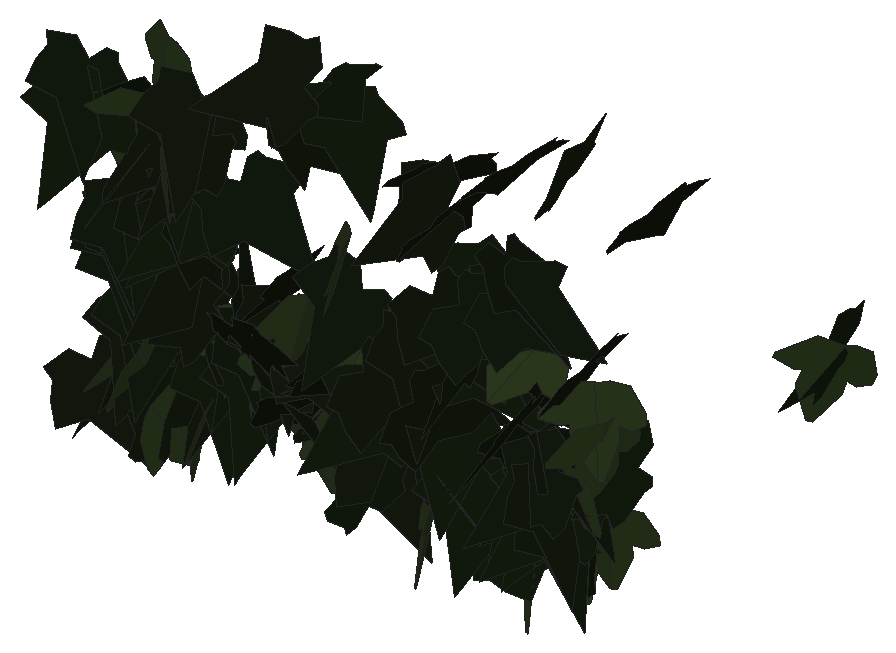
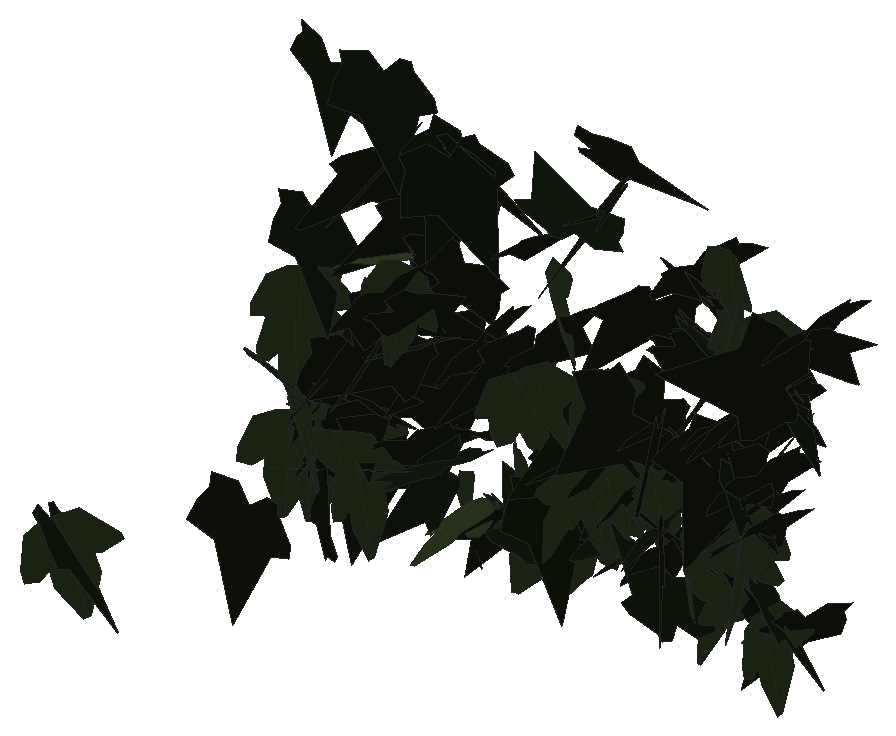
# SketchUp Ruby script. Lengths in inches.
U = 1.inch
M = Sketchup.active_model
def pt(a) = Geom::Point3d.new(a.map { |v| v * U })
def face(e, loops, mat)
  f = e.add_face(loops[0].map { |a| pt(a) })
  loops[1..].each { |l| e.add_face(l.map { |a| pt(a) }).erase! }
  f.material = f.back_material = mat if mat
  f
end
# faces: each face lists its corners as indices into pts; further lists are holes
def faces(e, pts, list, mat = nil) = list.each { |f| face(e, (f[0].is_a?(Array) ? f : [f]).map { |l| l.map { |i| pts[i] } }, mat) }
# xy, xz, yz: faces in a plane at the given z, y or x. An outline is a flat list of corners, or four numbers for a rectangle; further outlines are holes
def ring(l) = l.size == 4 ? [[l[0], l[1]], [l[2], l[1]], [l[2], l[3]], [l[0], l[3]]] : l.each_slice(2).to_a
def flat(e, list, mat, &to3) = list.each { |f| face(e, (f[0].is_a?(Array) ? f : [f]).map { |l| ring(l).map { |u, v| to3.(u, v) } }, mat) }
def xy(e, z, list, mat = nil) = flat(e, list, mat) { |x, y| [x, y, z] }
def xz(e, y, list, mat = nil) = flat(e, list, mat) { |x, z| [x, y, z] }
def yz(e, x, list, mat = nil) = flat(e, list, mat) { |y, z| [x, y, z] }
def lines(e, pts, list) = list.each { |a, b| e.add_line(pt(pts[a]), pt(pts[b])) }
# prism: a flat outline (further loops are holes) pulled along v
def prism(e, loops, v, mat = nil)
  f = face(e, loops, mat); d = Geom::Vector3d.new(v.map { |x| x * U })
  f.pushpull(f.normal.samedirection?(d) ? d.length : -d.length)
end
def box(e, o, s, mat = nil) = prism(e, [[o, [o[0] + s[0], o[1], o[2]], [o[0] + s[0], o[1] + s[1], o[2]], [o[0], o[1] + s[1], o[2]]]], [0, 0, s[2]], mat)
def at(x, y, z, deg = 0) = Geom::Transformation.translation(pt([x, y, z])) * Geom::Transformation.rotation(ORIGIN, Z_AXIS, deg.degrees)
def axes(o, x, y, z) = Geom::Transformation.new([*x, 0, *y, 0, *z, 0, *pt(o).to_a, 1])
def part(name) = M.definitions.add(name)
# library, detail: a bought-in or finely detailed component or shape, given as its bounding box
def library(name, o, s) = part(name).tap { |d| box(d.entities, o, s) }
def detail(e, o, s) = box(e.add_group.entities, o, s)
def put(e, d, t, mat = nil) = e.add_instance(d, t).tap { |i| i.material = mat if mat }
def group(e, t, mat = nil) = e.add_group.tap { |g| g.transformation = t; g.material = mat if mat }.entities
root = M.entities
M.materials.add("efeu1").color = [18, 25, 13]
M.materials.add("efeu2").color = [43, 57, 29]
c1 = part("ivyleaf_9")
p = [[1.54,2.16,1.25],[1.36,2.04,1.19],[-0.21,0.99,0.68],[-0.71,1.11,0.82],[-0.85,0.86,0.67],[-0.8,0.17,0.21],
  [-0.9,-0.01,0.1],[-0.67,-0.16,-0.02],[-0.08,-0.08,-0.05],[-0.03,-0.6,-0.4],[0.65,-0.88,-0.66],[0.83,-0.6,-0.49],
  [1.29,-0.42,-0.43],[1.8125,-0.07,-0.26],[1.21,0.44,0.15]]
faces(c1.entities,p,[[0,1,2,3,4,5,6,7,8,9,10,11,12,13,14]],"efeu1")
c2 = part("ivyleaf_10")
p = [[0,0.5,-0.03],[-0.0625,2.02,-0.43],[-0.19,2.01,-0.46],[-0.54,1.05,-0.29],[-0.52,0.625,-0.18],[-0.83,0.76,-0.28],
  [-1.16,0.64,-0.33],[-1.15,0.33,-0.24],[-0.77,-0.39,0.02],[-0.3,-0.51,0.16],[0.04,-0.48,0.23],[-0.02,2.01,-0.4375],
  [-0.06,2.01,-0.43],[0.04,-0.49,0.23],[0.67,-0.49,0.14],[1.38,0.36,-0.2],[1.375,0.51,-0.24],[0.81,0.65,-0.19],
  [0.62,0.59,-0.15],[0.6,1.09,-0.28],[0.5,1.23,-0.31]]
faces(c2.entities,p,[[0,1,2,3,4,5,6,7,8,9,10],[11,12,0,13,14,15,16,17,18,19,20]],"efeu2")
put(root,c1,axes([47.72,220.88,250.6],[0.48269,0.07432,-0.10717],[-0.10687,-0.01009,-0.48834],[-0.07475,0.49434,0.00615]))
put(root,c1,axes([45.87,221.22,251.43],[-0.28658,-0.25776,-0.31848],[0.28688,0.15125,-0.38056],[0.29252,-0.40085,0.0612]))
put(root,c1,axes([45.86,221,251.9],[-0.24087,0.43778,-0.01816],[0.00545,-0.01773,-0.49966],[-0.43813,-0.2409,0.00377]))
put(root,c1,axes([50.55,221.21,253.1],[-0.485,0.08676,0.08514],[-0.08165,0.02691,-0.49255],[-0.09005,-0.49168,-0.01194]))
put(root,c1,axes([46.95,221.31,252.72],[-0.48269,-0.01355,-0.12972],[0.13042,-0.04902,-0.4802],[0.0003,-0.49741,0.05086]))
put(root,c2,axes([51.67,221.51,251.4],[-0.46574,-0.06402,0.17026],[0.07904,-0.49274,0.03094],[0.16383,0.05573,0.4691]))
put(root,c1,axes([49.5,221.51,249.94],[-0.36577,-0.27031,0.2077],[-0.05758,-0.25128,-0.42842],[0.336,-0.33733,0.15269]))
put(root,c1,axes([46.99,221.38,251.82],[-0.44153,-0.19453,0.1312],[-0.12135,-0.04997,-0.48247],[0.20082,-0.45789,-0.00308]))
put(root,c1,axes([45.73,221.3,251.42],[0.00655,-0.49326,-0.08156],[0.00801,0.08166,-0.49322],[0.49989,0.00515,0.00897]))
put(root,c1,axes([46.98,221.36,251.88],[-0.47235,-0.15801,0.0438],[-0.04009,-0.01822,-0.49806],[0.15899,-0.47403,0.00454]))
put(root,c1,axes([48.35,221.25,253.93],[-0.43041,0.09578,0.23573],[-0.23974,0.00257,-0.43877],[-0.08526,-0.49073,0.04371]))
put(root,c1,axes([49.65,220.91,250.67],[0.16485,-0.15614,-0.44547],[-0.06723,0.45928,-0.18586],[0.46723,0.12118,0.13043]))
put(root,c1,axes([45.18,221.45,252.5625],[-0.36804,-0.33837,-0.00719],[0.04169,-0.03479,-0.49704],[0.33586,-0.36647,0.05382]))
put(root,c1,axes([51.73,220.97,252.44],[0.14388,-0.19734,-0.4363],[0.02441,0.458,-0.19911],[0.47823,0.03599,0.14142]))
put(root,c1,axes([46.7,221.46,253.0625],[-0.15688,-0.47475,-0.00186],[0.0095,-0.00118,-0.49991],[0.47466,-0.15689,0.00939]))
put(root,c1,axes([51.03,220.99,252.02],[0.14519,-0.1569,-0.452],[0.0491,0.47474,-0.14902],[0.47593,-0.00112,0.15326]))
put(root,c1,axes([52.08,221.38,249.99],[-0.49806,-0.01387,0.04179],[-0.04175,-0.00196,-0.49825],[0.01399,-0.4998,0.00079]))
put(root,c2,axes([46.12,221.06,249.6],[-0.02409,-0.41286,-0.281],[0.00436,0.28115,-0.41345],[0.4994,-0.02237,-0.00994]))
put(root,c1,axes([48.98,221.59,251.24],[-0.16849,-0.42915,0.19349],[-0.07482,-0.17848,-0.46103],[0.46477,-0.18431,-0.00407]))
put(root,c1,axes([50.9375,221.35,251.47],[-0.4113,0.16437,-0.23198],[0.21353,-0.09077,-0.44291],[-0.18772,-0.4634,0.00447]))
put(root,c1,axes([46.63,221.65,250.62],[-0.19007,-0.33267,0.32125],[-0.15673,-0.28044,-0.38313],[0.4351,-0.24634,0.00233]))
put(root,c1,axes([51.63,221.4375,250.67],[-0.30725,0.22014,-0.32731],[0.16141,-0.3084,-0.35894],[-0.35992,-0.32623,0.11845]))
put(root,c2,axes([48.91,221.34,251.89],[0.27058,-0.41982,0.02312],[0.01249,-0.01945,-0.49947],[0.42027,0.27087,-0.00003]))
put(root,c2,axes([46.51,221.1,252.3],[-0.21046,0.42452,0.15966],[-0.13078,0.11174,-0.46948],[-0.43428,-0.23938,0.06401]))
put(root,c1,axes([51.48,221.27,252.69],[0.28969,-0.3867,-0.1286],[-0.02866,0.13806,-0.47971],[0.40652,0.28531,0.05782]))
put(root,c1,axes([49.94,221.53,250.91],[0.01978,-0.49613,0.05885],[-0.00519,-0.05909,-0.49647],[0.49958,0.01903,-0.00749]))
put(root,c1,axes([50.39,220.92,250.55],[0.0597,0.02583,-0.49575],[-0.12247,0.48465,0.0105],[0.48108,0.12018,0.0642]))
put(root,c1,axes([46.37,221.41,252.52],[-0.48877,0.1053,0.00367],[-0.00316,0.00274,-0.49998],[-0.10531,-0.48878,-0.00202]))
put(root,c1,axes([46.93,221.34,250.46],[-0.43618,0.20953,0.12586],[-0.12113,0.03833,-0.48359],[-0.2123,-0.45236,0.01732]))
put(root,c1,axes([45.83,221.66,249.78],[-0.16359,-0.46129,0.10224],[0.01178,-0.11215,-0.48712],[0.47234,-0.15696,0.04756]))
put(root,c1,axes([47.71,221.54,249.85],[-0.39343,-0.25545,-0.17307],[0.16834,0.05734,-0.4673],[0.25859,-0.42598,0.04089]))
put(root,c1,axes([44.9,221.6,252.89],[-0.04695,-0.4969,0.02974],[0.04141,-0.03367,-0.49714],[0.49607,-0.04421,0.04431]))
put(root,c1,axes([50.34,221.32,251.74],[-0.07025,-0.18548,-0.45898],[0.3477,0.3115,-0.1791],[0.35238,-0.34433,0.08521]))
put(root,c1,axes([45.89,221.64,249.96],[-0.07804,-0.48826,0.07427],[-0.00214,-0.07485,-0.49436],[0.49387,-0.07748,0.0096]))
put(root,c2,axes([48.18,221.52,250.74],[-0.05434,-0.47907,0.13244],[0.0418,-0.13716,-0.479],[0.49528,-0.04098,0.05496]))
put(root,c1,axes([50.55,221.02,252.93],[0.11115,0.45339,0.17912],[0.00761,0.18208,-0.46561],[-0.48743,0.10623,0.03358]))
put(root,c1,axes([50.44,221.57,250.11],[-0.22611,-0.42559,-0.13322],[0.04662,0.126,-0.48161],[0.44351,-0.23021,-0.0173]))
put(root,c1,axes([51.89,221.57,249.65],[0.07843,-0.49031,-0.0587],[-0.00535,0.05859,-0.49653],[0.49378,0.07851,0.00395]))
put(root,c1,axes([46.42,221.22,248.73],[-0.15528,0.20824,0.42723],[-0.30211,0.30372,-0.25784],[-0.3669,-0.33822,0.0315]))
put(root,c1,axes([50.83,221.69,249.34],[-0.24301,-0.43623,-0.02544],[0.06362,-0.00652,-0.49589],[0.43232,-0.24425,0.05867]))
put(root,c1,axes([47.75,221.56,249.72],[0.27628,-0.37675,0.17813],[0.15625,-0.10449,-0.46332],[0.38634,0.31168,0.06]))
put(root,c1,axes([45.37,221.57,251.02],[0.19795,-0.45898,0.01221],[0.00412,-0.01152,-0.49985],[0.45913,0.19799,-0.00078]))
put(root,c2,axes([51.61,221.53,248.74],[0.3515,-0.33989,0.10453],[0.12567,-0.01876,-0.48358],[0.33265,0.36623,0.07225]))
put(root,c2,axes([46.77,221.47,248.89],[0.21955,-0.44444,-0.06537],[-0.01561,0.06517,-0.49549],[0.44895,0.21961,0.01474]))
put(root,c1,axes([47.44,221.35,252.24],[0.05076,-0.30353,-0.39408],[0.06457,0.39679,-0.2973],[0.49321,-0.02071,0.07947]))
put(root,c1,axes([48.33,221.17,249.82],[0.23085,0.44184,0.03853],[0.01586,0.03518,-0.49851],[-0.44323,0.23139,0.00222]))
put(root,c2,axes([46.36,221.1875,248.8],[0.03236,0.39242,0.30815],[-0.0895,0.30835,-0.38329],[-0.49086,-0.03036,0.0902]))
put(root,c2,axes([50.02,221.64,248.75],[0.30302,-0.3628,0.16296],[0.11711,-0.11439,-0.47244],[0.38008,0.32449,0.01565]))
put(root,c1,axes([45.97,221.7,251.37],[0.05841,-0.49658,-0.0001],[-0.00304,-0.00025,-0.49999],[0.49657,0.05841,-0.00305]))
put(root,c1,axes([52.0625,221.76,249.47],[-0.43554,-0.21789,0.11326],[-0.09994,-0.05336,-0.487],[0.22431,-0.44685,0.00293]))
put(root,c1,axes([46.04,221.62,250.65],[-0.33043,0.22102,-0.30325],[0.25787,-0.1598,-0.39745],[-0.27261,-0.41906,-0.00839]))
put(root,c2,axes([47.63,221.78,249.83],[-0.00924,-0.39775,0.30284],[0.14845,-0.29141,-0.37821],[0.47736,0.08293,0.12348]))
put(root,c1,axes([45.59,221.71,250.72],[-0.06487,-0.49065,-0.07107],[-0.00085,0.07179,-0.49482],[0.49577,-0.06407,-0.01015]))
put(root,c1,axes([52.55,221.29,251.56],[-0.08745,0.49086,0.03753],[-0.00572,0.0371,-0.49859],[-0.49226,-0.08763,-0.00087]))
put(root,c1,axes([48.08,221.28,253.41],[0.36115,-0.11351,-0.32663],[-0.22752,0.27765,-0.34806],[0.2604,0.40003,0.14889]))
put(root,c1,axes([47.33,221.73,250.04],[0.09948,-0.49,0.0028],[0.00003,-0.00285,-0.49999],[0.49,0.09948,-0.00054]))
put(root,c1,axes([46.54,221.41,251.39],[0.3392,-0.27471,-0.24388],[-0.13298,0.21761,-0.43007],[0.34243,0.35662,0.07456]))
put(root,c1,axes([45.04,221.54,248.92],[0.08641,-0.39692,-0.29152],[0.04731,0.3013,-0.39621],[0.4902,0.04089,0.08963]))
put(root,c1,axes([51.45,221.38,253.9],[-0.00701,0.49978,-0.01312],[-0.08373,-0.01411,-0.49274],[-0.49289,-0.00471,0.08389]))
put(root,c1,axes([46.89,221.84,249.59],[-0.42561,-0.1282,-0.22895],[0.2488,-0.05854,-0.42973],[0.08338,-0.47973,0.11363]))
put(root,c1,axes([46.54,221.71,252.36],[-0.46065,0.18843,-0.04794],[0.01566,-0.08693,-0.49214],[-0.1938,-0.4549,0.07419]))
put(root,c2,axes([45.66,221.68,252.54],[-0.3423,-0.34468,0.11846],[-0.08966,-0.07788,-0.48569],[0.35326,-0.35374,-0.0085]))
put(root,c1,axes([48.35,221.22,249.9375],[0.29302,0.25352,0.31602],[0.12,0.3182,-0.36653],[-0.38697,0.29065,0.12563]))
put(root,c1,axes([45.52,221.71,249.22],[-0.41247,0.23568,-0.15597],[0.13414,-0.07962,-0.47504],[-0.24875,-0.43372,0.00245]))
put(root,c1,axes([46.8125,221.85,249.44],[-0.01513,-0.49914,-0.02507],[-0.00077,0.0251,-0.49937],[0.49977,-0.01507,-0.00153]))
put(root,c1,axes([51.78,221.78,249.2],[0.13095,-0.47879,-0.0601],[-0.00935,0.05974,-0.49633],[0.48246,0.13111,0.00669]))
put(root,c2,axes([47.11,221.67,250.08],[0.48518,0.11798,0.02613],[0.02061,0.02573,-0.49891],[-0.11906,0.4852,0.02011]))
put(root,c1,axes([51.56,221.92,249.77],[-0.43659,-0.20691,-0.12875],[0.16786,-0.06383,-0.46664],[0.17667,-0.45068,0.1252]))
put(root,c2,axes([51.76,221.6875,249.39],[-0.39457,-0.30379,0.045],[-0.02939,-0.03558,-0.49787],[0.3057,-0.39553,0.01022]))
put(root,c1,axes([50.34,221.61,249.05],[0.45863,-0.1956,-0.03742],[-0.03349,0.01686,-0.49859],[0.19631,0.45984,0.00236]))
put(root,c2,axes([52.41,221.76,250.92],[-0.39866,-0.30173,0.00481],[0.09407,-0.13183,-0.47304],[0.28673,-0.37627,0.16188]))
put(root,c2,axes([49.06,221.78,250.6],[-0.3633,-0.16745,0.29996],[-0.24958,-0.17134,-0.39793],[0.23606,-0.43887,0.04092]))
put(root,c1,axes([47.6,221.88,250.36],[0.01717,-0.49873,-0.03123],[-0.00649,0.03102,-0.49899],[0.49966,0.01754,-0.0054]))
put(root,c2,axes([45.99,221.76,252.74],[-0.29298,0.36276,-0.18046],[0.09972,-0.15128,-0.46601],[-0.39271,-0.30906,0.01629]))
put(root,c2,axes([49.03,221.8,250.78],[0.36735,0.2808,-0.19028],[-0.1721,-0.08741,-0.46124],[-0.2923,0.40436,0.03243]))
put(root,c1,axes([48.125,221.76,250.13],[0.15825,-0.44082,-0.17503],[0.10615,0.21275,-0.43985],[0.46227,0.10205,0.16092]))
put(root,c2,axes([46.02,221.74,253.35],[-0.44706,0.21175,0.07278],[-0.1291,-0.11099,-0.47012],[-0.18294,-0.43914,0.15391]))
put(root,c1,axes([51.61,221.64,250.16],[0.24324,0.34277,-0.27082],[-0.15029,-0.22539,-0.42025],[-0.41018,0.28584,-0.00662]))
put(root,c1,axes([51.77,222.02,249.4375],[-0.35193,-0.35314,0.03796],[-0.02529,-0.02838,-0.49855],[0.35427,-0.35283,0.00212]))
put(root,c1,axes([49.23,221.45,248.58],[0.05062,0.29666,0.39929],[-0.26452,0.35595,-0.23092],[-0.42127,-0.18786,0.19298]))
put(root,c2,axes([51.99,221.69,249.66],[0.47724,-0.0284,-0.14641],[-0.13033,0.15916,-0.45572],[0.07249,0.47314,0.14451]))
put(root,c2,axes([48.17,221.73,249.22],[-0.49332,0.05482,-0.06023],[0.05676,-0.03374,-0.49562],[-0.0584,-0.49584,0.02707]))
put(root,c2,axes([52.46,221.77,250.44],[-0.19485,-0.45938,-0.03165],[0.02032,0.02576,-0.49892],[0.46002,-0.19572,0.00863]))
put(root,c1,axes([50.2,221.69,253.3125],[-0.02339,0.44878,-0.21919],[-0.13618,-0.21685,-0.42945],[-0.48053,0.03961,0.13238]))
put(root,c1,axes([51.18,221.54,248.74],[0.42904,-0.17752,-0.1855],[0.13537,0.46335,-0.13032],[0.21817,0.0616,0.44565]))
put(root,c2,axes([46.07,221.88,249.92],[0.27692,0.2268,-0.34911],[-0.34436,-0.11084,-0.34516],[-0.23395,0.4316,0.09481]))
put(root,c2,axes([45.78,221.78,249.52],[0.19066,-0.46026,-0.0425],[0.14341,0.10261,-0.46787],[0.43941,0.16622,0.17114]))
put(root,c1,axes([50.4375,221.82,250.86],[0.21179,-0.43284,-0.13339],[0.22332,0.2279,-0.38495],[0.39405,0.10348,0.28986]))
put(root,c1,axes([51.48,221.5625,249.05],[0.15717,0.47372,-0.02984],[-0.01456,-0.02661,-0.49908],[-0.47443,0.15775,0.00543]))
put(root,c1,axes([49.09,221.86,249.07],[0.06305,-0.43298,-0.24197],[0.06066,0.24882,-0.42943],[0.49229,0.0248,0.08391]))
put(root,c1,axes([46.09,221.59,250.79],[0.31764,0.38429,-0.03778],[-0.03061,-0.0237,-0.4985],[-0.38492,0.319,0.00847]))
put(root,c1,axes([50.16,221.9,249.32],[0.21211,-0.44488,-0.08421],[0.22447,0.18408,-0.4071],[0.39322,0.13489,0.27781]))
put(root,c1,axes([47.24,221.73,250.06],[0.01619,-0.28752,0.40874],[0.03591,0.40857,0.28597],[-0.49845,0.0201,0.03388]))
put(root,c1,axes([51.8,221.95,249.98],[0.21477,-0.44327,-0.08594],[0.00458,0.0973,-0.49042],[0.4515,0.20987,0.04586]))
put(root,c1,axes([50.86,221.6875,250.76],[0.47511,0.08605,0.12985],[0.12889,0.01696,-0.48281],[-0.0875,0.49225,-0.00607]))
put(root,c1,axes([52.125,221.56,253.89],[-0.07942,0.40067,0.28836],[-0.07811,0.27819,-0.40805],[-0.48743,-0.10986,0.01841]))
put(root,c1,axes([46.79,221.91,249.75],[0.30422,-0.38642,-0.09016],[0.03498,0.13928,-0.47894],[0.39526,0.28509,0.11177]))
put(root,c2,axes([45.23,221.97,248.87],[-0.02536,-0.49928,0.0086],[-0.00058,-0.00858,-0.49993],[0.49936,-0.02536,-0.00014]))
put(root,c2,axes([47.95,222,249.92],[-0.38117,-0.14687,0.28835],[-0.24579,-0.1584,-0.40558],[0.21048,-0.45093,0.04855]))
put(root,c2,axes([49.01,221.89,249.72],[0.3428,-0.34644,-0.11165],[0.00669,0.15934,-0.47388],[0.36393,0.3234,0.11388]))
put(root,c2,axes([48.57,221.93,249.16],[-0.37635,-0.2893,-0.15706],[0.19441,-0.00283,-0.46065],[0.26564,-0.4078,0.11462]))
put(root,c1,axes([47.97,222.17,253.42],[0.01295,-0.49551,-0.06558],[0.48781,0.02684,-0.10642],[0.10898,-0.06123,0.48412]))
put(root,c1,axes([47.67,221.53,250.74],[0.17957,0.30882,0.34984],[0.10416,0.33886,-0.3526],[-0.45487,0.19951,0.05736]))
put(root,c1,axes([48.32,222.18,249.04],[0.01279,-0.48878,0.10456],[0.47438,-0.02108,-0.15658],[0.15747,0.10321,0.4632]))
put(root,c1,axes([52.68,222.11,249.94],[-0.47715,0.14616,0.03111],[-0.0578,-0.0845,-0.48941],[-0.1378,-0.47064,0.09753]))
put(root,c2,axes([51.71,221.91,248.93],[0.28766,0.36938,0.17553],[0.11967,0.12918,-0.46797],[-0.39106,0.31124,-0.01408]))
put(root,c1,axes([48.31,222.21,253.25],[-0.01448,-0.4951,-0.06833],[0.14491,0.06126,-0.4746],[0.47832,-0.03355,0.14171]))
put(root,c2,axes([51.25,222.08,248.91],[-0.07208,-0.49473,0.00665],[-0.00435,-0.00608,-0.49994],[0.49476,-0.07213,-0.00343]))
put(root,c1,axes([46.53,222.09,248.64],[0.17188,-0.45567,0.11324],[0.46016,0.18744,0.05582],[-0.09333,0.08503,0.4838]))
put(root,c1,axes([50.47,222.34,251.5],[-0.40914,-0.21733,0.18808],[-0.15182,-0.11441,-0.46245],[0.24405,-0.43552,0.02763]))
put(root,c2,axes([50.66,222.01,251.63],[-0.49333,0.08098,-0.00836],[0.0048,-0.02231,-0.49948],[-0.08127,-0.49289,0.02123]))
put(root,c1,axes([45.12,221.87,252.18],[0.28512,-0.00579,0.4107],[0.39341,0.14755,-0.27103],[-0.11806,0.4777,0.08869]))
put(root,c2,axes([52.34,222.09,249.12],[-0.44128,-0.23412,0.02146],[-0.01834,-0.01123,-0.49954],[0.23438,-0.44166,0.00132]))
put(root,c2,axes([51.49,222.16,249.28],[0.46563,0.17966,-0.03022],[-0.02411,-0.02143,-0.49896],[-0.18058,0.46611,-0.01129]))
put(root,c1,axes([50.74,222.3,251.625],[-0.00297,-0.48505,-0.1213],[-0.00671,0.12133,-0.48501],[0.49995,-0.00125,-0.00723]))
put(root,c2,axes([51.83,222.04,249.37],[0.13651,-0.43131,-0.21293],[0.04881,0.23262,-0.43989],[0.47852,0.09931,0.10562]))
put(root,c1,axes([50.83,222.25,250.91],[0.29737,-0.39045,-0.09549],[-0.07314,0.06423,-0.49043],[0.39525,0.30565,-0.01891]))
put(root,c1,axes([48.42,222.07,249.52],[-0.07277,0.49465,0.00529],[-0.00125,0.00517,-0.49997],[-0.49467,-0.07278,0.00049]))
put(root,c2,axes([48.03,222.04,249.93],[-0.02497,0.42307,0.2653],[-0.06657,0.26044,-0.42159],[-0.49492,-0.05638,0.04332]))
put(root,c2,axes([52.12,222.16,249.45],[0.17689,-0.22478,-0.4101],[-0.2603,0.31694,-0.286],[0.38853,0.31468,-0.00489]))
put(root,c2,axes([49.65,222.02,248.93],[0.43349,-0.11397,-0.22158],[0.1053,0.48677,-0.04436],[0.22583,-0.0082,0.44602]))
put(root,c1,axes([46.68,222.15,249.82],[0.07253,-0.03712,-0.49332],[-0.46646,0.16095,-0.08069],[0.16479,0.47193,-0.01128]))
put(root,c1,axes([51.78,222.22,248.17],[0.16362,-0.11168,0.45908],[-0.13517,0.45446,0.15872],[-0.45272,-0.17605,0.11852]))
put(root,c2,axes([52.4,226.27,249.52],[-0.32789,-0.33682,0.1704],[-0.12287,-0.11818,-0.47004],[0.35692,-0.35012,-0.00527]))
put(root,c1,axes([49.83,225.97,250.66],[0.04766,0.49,0.08732],[-0.01361,0.08897,-0.49183],[-0.49754,0.0445,0.02182]))
put(root,c1,axes([52.47,226.28,249.67],[-0.37361,0.3273,-0.05734],[0.04008,-0.04127,-0.49668],[-0.32986,-0.37573,0.0046]))
